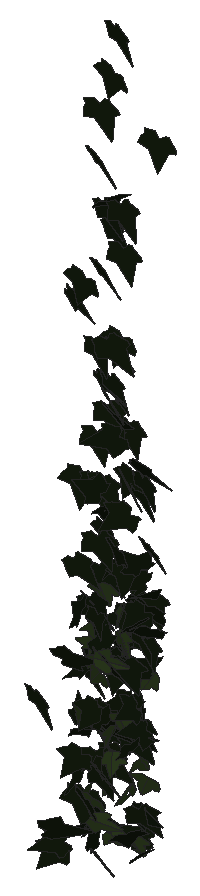
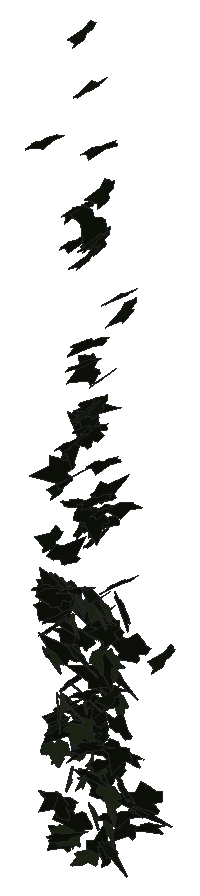
# SketchUp Ruby script. Lengths in inches.
U = 1.inch
M = Sketchup.active_model
def pt(a) = Geom::Point3d.new(a.map { |v| v * U })
def face(e, loops, mat)
  f = e.add_face(loops[0].map { |a| pt(a) })
  loops[1..].each { |l| e.add_face(l.map { |a| pt(a) }).erase! }
  f.material = f.back_material = mat if mat
  f
end
# faces: each face lists its corners as indices into pts; further lists are holes
def faces(e, pts, list, mat = nil) = list.each { |f| face(e, (f[0].is_a?(Array) ? f : [f]).map { |l| l.map { |i| pts[i] } }, mat) }
# xy, xz, yz: faces in a plane at the given z, y or x. An outline is a flat list of corners, or four numbers for a rectangle; further outlines are holes
def ring(l) = l.size == 4 ? [[l[0], l[1]], [l[2], l[1]], [l[2], l[3]], [l[0], l[3]]] : l.each_slice(2).to_a
def flat(e, list, mat, &to3) = list.each { |f| face(e, (f[0].is_a?(Array) ? f : [f]).map { |l| ring(l).map { |u, v| to3.(u, v) } }, mat) }
def xy(e, z, list, mat = nil) = flat(e, list, mat) { |x, y| [x, y, z] }
def xz(e, y, list, mat = nil) = flat(e, list, mat) { |x, z| [x, y, z] }
def yz(e, x, list, mat = nil) = flat(e, list, mat) { |y, z| [x, y, z] }
def lines(e, pts, list) = list.each { |a, b| e.add_line(pt(pts[a]), pt(pts[b])) }
# prism: a flat outline (further loops are holes) pulled along v
def prism(e, loops, v, mat = nil)
  f = face(e, loops, mat); d = Geom::Vector3d.new(v.map { |x| x * U })
  f.pushpull(f.normal.samedirection?(d) ? d.length : -d.length)
end
def box(e, o, s, mat = nil) = prism(e, [[o, [o[0] + s[0], o[1], o[2]], [o[0] + s[0], o[1] + s[1], o[2]], [o[0], o[1] + s[1], o[2]]]], [0, 0, s[2]], mat)
def at(x, y, z, deg = 0) = Geom::Transformation.translation(pt([x, y, z])) * Geom::Transformation.rotation(ORIGIN, Z_AXIS, deg.degrees)
def axes(o, x, y, z) = Geom::Transformation.new([*x, 0, *y, 0, *z, 0, *pt(o).to_a, 1])
def part(name) = M.definitions.add(name)
# library, detail: a bought-in or finely detailed component or shape, given as its bounding box
def library(name, o, s) = part(name).tap { |d| box(d.entities, o, s) }
def detail(e, o, s) = box(e.add_group.entities, o, s)
def put(e, d, t, mat = nil) = e.add_instance(d, t).tap { |i| i.material = mat if mat }
def group(e, t, mat = nil) = e.add_group.tap { |g| g.transformation = t; g.material = mat if mat }.entities
root = M.entities
M.materials.add("1026 AP 7946 SUNNY SIDE UP").color = [254, 231, 186]
M.materials.add("efeu1").color = [18, 25, 13]
M.materials.add("efeu2").color = [43, 57, 29]
c1 = part("ivyleaf_9")
p = [[1.54,2.16,1.25],[1.36,2.04,1.19],[-0.21,0.99,0.68],[-0.71,1.11,0.82],[-0.85,0.86,0.67],[-0.8,0.17,0.21],
  [-0.9,-0.01,0.1],[-0.67,-0.16,-0.02],[-0.08,-0.08,-0.05],[-0.03,-0.6,-0.4],[0.65,-0.88,-0.66],[0.83,-0.6,-0.49],
  [1.29,-0.42,-0.43],[1.8125,-0.07,-0.26],[1.21,0.44,0.15]]
faces(c1.entities,p,[[0,1,2,3,4,5,6,7,8,9,10,11,12,13,14]],"efeu1")
c2 = part("ivyleaf_10")
p = [[0,0.5,-0.03],[-0.0625,2.02,-0.43],[-0.19,2.01,-0.46],[-0.54,1.05,-0.29],[-0.52,0.625,-0.18],[-0.83,0.76,-0.28],
  [-1.16,0.64,-0.33],[-1.15,0.33,-0.24],[-0.77,-0.39,0.02],[-0.3,-0.51,0.16],[0.04,-0.48,0.23],[-0.02,2.01,-0.4375],
  [-0.06,2.01,-0.43],[0.04,-0.49,0.23],[0.67,-0.49,0.14],[1.38,0.36,-0.2],[1.375,0.51,-0.24],[0.81,0.65,-0.19],
  [0.62,0.59,-0.15],[0.6,1.09,-0.28],[0.5,1.23,-0.31]]
faces(c2.entities,p,[[0,1,2,3,4,5,6,7,8,9,10],[11,12,0,13,14,15,16,17,18,19,20]],"efeu2")
put(root,c1,axes([148.02,211.49,307.71],[-0.3468,-0.39947,-0.07155],[0.08263,0.04763,-0.46923],[0.63156,-0.22559,0.0221]),"1026 AP 7946 SUNNY SIDE UP")
put(root,c1,axes([148.12,211.17,296.1],[0.2283,0.3421,0.04637],[0.05922,0.03071,-0.38197],[-0.53891,0.1483,-0.02233]),"1026 AP 7946 SUNNY SIDE UP")
put(root,c1,axes([148.43,211.57,291.55],[-0.32957,0.32893,-0.01711],[-0.01222,-0.02684,-0.40138],[-0.51788,-0.20869,0.02037]),"1026 AP 7946 SUNNY SIDE UP")
put(root,c1,axes([148.27,210.93,294.23],[-0.39626,0.1337,-0.24009],[0.2906,-0.14709,-0.29271],[-0.30808,-0.31071,0.0327]),"1026 AP 7946 SUNNY SIDE UP")
put(root,c1,axes([148.47,211.86,300.53],[0.2781,-0.0272,-0.37505],[-0.57357,-0.02467,-0.18088],[-0.0163,0.40385,-0.03393]),"1026 AP 7946 SUNNY SIDE UP")
put(root,c2,axes([148.45,211.59,292.53],[0.30772,-0.23415,-0.22991],[-0.18469,0.18993,-0.31216],[0.47236,0.2268,0.02772]),"1026 AP 7946 SUNNY SIDE UP")
put(root,c1,axes([148.4,210.83,296.7],[0.37132,-0.08,0.31455],[-0.19132,0.32929,0.18747],[-0.45871,-0.2021,0.17644]),"1026 AP 7946 SUNNY SIDE UP")
put(root,c1,axes([148.01,210.98,303.96],[0.22055,-0.35797,-0.20662],[0.04313,0.21761,-0.38299],[0.64221,0.10832,0.09668]),"1026 AP 7946 SUNNY SIDE UP")
put(root,c1,axes([148.04,210.58,316.57],[0.50068,-0.29251,-0.15557],[-0.13487,0.12673,-0.44336],[0.4985,0.32807,0.03629]),"1026 AP 7946 SUNNY SIDE UP")
put(root,c1,axes([148.23,211.31,293.03],[-0.31586,-0.4262,-0.08847],[0.07842,0.0687,-0.48472],[0.67836,-0.20639,0.01484]),"1026 AP 7946 SUNNY SIDE UP")
put(root,c1,axes([148.49,209.25,291.48],[-0.43927,-0.24623,0.10603],[-0.08854,-0.09332,-0.38279],[0.41105,-0.28323,0.03085]),"1026 AP 7946 SUNNY SIDE UP")
put(root,c2,axes([148.43,211.375,293.48],[0.06296,-0.38932,-0.05728],[-0.0047,0.05337,-0.40287],[0.61788,0.04008,0.00277]),"1026 AP 7946 SUNNY SIDE UP")
put(root,c1,axes([148.67,210.84,299.35],[-0.45934,0.25194,-0.06801],[0.0441,-0.07034,-0.39623],[-0.40772,-0.29144,0.03376]),"1026 AP 7946 SUNNY SIDE UP")
put(root,c2,axes([148.47,211.86,300.69],[-0.37739,-0.31995,-0.0014],[0.04429,-0.02169,-0.41054],[0.50114,-0.23902,0.03522]),"1026 AP 7946 SUNNY SIDE UP")
put(root,c2,axes([148.64,211.45,300.1],[-0.54408,-0.13297,0.1484],[-0.16304,-0.12561,-0.37481],[0.26264,-0.35344,0.07475]),"1026 AP 7946 SUNNY SIDE UP")
put(root,c1,axes([148.86,209.05,292],[-0.57488,-0.00113,0.14571],[-0.22122,-0.03782,-0.37515],[0.02311,-0.39019,0.03363]),"1026 AP 7946 SUNNY SIDE UP")
put(root,c1,axes([148.14,211.56,298.66],[0.31074,-0.32465,0.07864],[0.04766,-0.07303,-0.39178],[0.52291,0.19958,-0.01103]),"1026 AP 7946 SUNNY SIDE UP")
put(root,c1,axes([148.04,211.73,301.84],[0.48195,-0.28561,0.13461],[0.11778,-0.11316,-0.43113],[0.4807,0.31407,-0.02933]),"1026 AP 7946 SUNNY SIDE UP")
put(root,c1,axes([148.12,208.23,298.98],[0.28091,-0.42459,0.1275],[0.05226,-0.12281,-0.47497],[0.69452,0.18097,-0.01583]),"1026 AP 7946 SUNNY SIDE UP")
put(root,c1,axes([148.375,211.09,317.13],[-0.20298,-0.3874,0.21408],[0.03188,-0.22382,-0.41382],[0.69215,-0.1033,0.08184]),"1026 AP 7946 SUNNY SIDE UP")
put(root,c1,axes([148.92,210.14,302.25],[-0.23648,0.02892,-0.46874],[-0.62543,0.2262,0.15152],[0.35092,0.42265,-0.04583]),"1026 AP 7946 SUNNY SIDE UP")
put(root,c2,axes([148.49,212.05,302.71],[0.39773,-0.28468,0.10174],[0.07112,-0.09374,-0.39184],[0.46929,0.25548,-0.02684]),"1026 AP 7946 SUNNY SIDE UP")
put(root,c1,axes([148.7,210.41,295.41],[-0.5666,-0.15043,-0.03454],[0.067,-0.01755,-0.40097],[0.2326,-0.36139,0.03137]),"1026 AP 7946 SUNNY SIDE UP")
put(root,c1,axes([148.33,211.75,307.58],[0.03559,-0.4106,-0.0915],[0.02211,0.0873,-0.42271],[0.65943,0.01924,0.01911]),"1026 AP 7946 SUNNY SIDE UP")
put(root,c1,axes([148.53,210.09,291.93],[0.20788,0.26926,0.22379],[0.1634,0.1892,-0.3078],[-0.51729,0.16796,-0.00729]),"1026 AP 7946 SUNNY SIDE UP")
put(root,c1,axes([148.2,211.9,322.52],[0.44796,-0.35322,0.0717],[0.02404,-0.07935,-0.46636],[0.56619,0.28283,-0.03693]),"1026 AP 7946 SUNNY SIDE UP")
put(root,c1,axes([148.38,212.125,324.74],[-0.01978,-0.45164,-0.12101],[0.04719,0.11392,-0.46401],[0.73125,-0.01957,0.02667]),"1026 AP 7946 SUNNY SIDE UP")
put(root,c1,axes([148.41,211.82,313.78],[0.1123,-0.43319,0.01438],[0.00141,-0.01649,-0.45239],[0.68164,0.0714,-0.00144]),"1026 AP 7946 SUNNY SIDE UP")
put(root,c1,axes([148.53,211.73,309.71],[-0.0936,-0.40561,-0.11167],[0.04233,0.10324,-0.42157],[0.65788,-0.06435,0.01124]),"1026 AP 7946 SUNNY SIDE UP")
put(root,c1,axes([148.7,211.13,290.84],[-0.03648,-0.08423,0.40935],[0.30326,0.34853,0.08965],[-0.56292,0.19322,0.02177]),"1026 AP 7946 SUNNY SIDE UP")
put(root,c1,axes([149.03,211.98,303.47],[-0.33954,0.33116,-0.0353],[0.00291,-0.04188,-0.40694],[-0.5238,-0.2149,0.02062]),"1026 AP 7946 SUNNY SIDE UP")
put(root,c1,axes([148.59,211.9,300.75],[-0.07609,-0.30763,0.28979],[-0.01236,-0.28421,-0.32128],[0.6572,-0.04097,0.02751]),"1026 AP 7946 SUNNY SIDE UP")
put(root,c2,axes([148.83,212.08,293.39],[0.33532,-0.28954,-0.11551],[-0.07935,0.09988,-0.36942],[0.48079,0.21842,0.01959]),"1026 AP 7946 SUNNY SIDE UP")
put(root,c1,axes([148.43,211.45,302.08],[-0.18706,-0.13328,-0.39864],[0.59372,0.11774,-0.16099],[0.24532,-0.38657,0.08566]),"1026 AP 7946 SUNNY SIDE UP")
put(root,c1,axes([148.3,209.87,299.98],[0.14046,-0.07305,0.42356],[0.61345,-0.13649,-0.11299],[0.23591,0.39841,0.04163]),"1026 AP 7946 SUNNY SIDE UP")
put(root,c1,axes([148.31,208.85,292.45],[0.31391,0.07645,0.44212],[0.6705,0.06146,-0.21549],[-0.13906,0.46892,-0.04098]),"1026 AP 7946 SUNNY SIDE UP")
put(root,c1,axes([148.57,211.99,303.38],[0.26727,-0.34837,-0.19096],[-0.02463,0.1936,-0.39271],[0.61855,0.15824,0.06687]),"1026 AP 7946 SUNNY SIDE UP")
put(root,c2,axes([149.08,210.0625,297.63],[-0.52109,0.16773,0.13464],[-0.21786,0.01096,-0.37912],[-0.25242,-0.35572,0.04926]),"1026 AP 7946 SUNNY SIDE UP")
put(root,c1,axes([149.17,212.4,296.32],[-0.40869,-0.17373,0.29317],[-0.32956,-0.19708,-0.3212],[0.40943,-0.33206,0.03409]),"1026 AP 7946 SUNNY SIDE UP")
put(root,c2,axes([148.87,211.61,302.76],[-0.60877,0.00636,-0.08419],[0.12702,-0.03828,-0.39738],[-0.02218,-0.39384,0.03494]),"1026 AP 7946 SUNNY SIDE UP")
put(root,c1,axes([148.62,212.07,320.23],[0.27941,-0.42204,-0.05816],[-0.01888,0.05359,-0.47133],[0.66877,0.17784,0.01099]),"1026 AP 7946 SUNNY SIDE UP")
put(root,c1,axes([148.61,211.81,312.36],[0.47341,-0.29564,-0.08159],[-0.0395,0.08451,-0.43205],[0.47895,0.29919,0.04501]),"1026 AP 7946 SUNNY SIDE UP")
put(root,c1,axes([149.21,210.97,307.52],[-0.0249,0.05717,0.46104],[-0.5437,-0.28869,0.02372],[0.4549,-0.34191,0.05358]),"1026 AP 7946 SUNNY SIDE UP")
put(root,c1,axes([148.58,211.58,299.46],[0.12732,0.0256,0.43926],[0.64664,0.11213,-0.08677],[-0.18077,0.41913,-0.00098]),"1026 AP 7946 SUNNY SIDE UP")
put(root,c1,axes([149.33,212.03,294.95],[-0.5707,-0.01598,0.0646],[-0.0965,-0.0299,-0.37342],[0.03271,-0.36712,0.02544]),"1026 AP 7946 SUNNY SIDE UP")
put(root,c2,axes([148.98,210.74,300.01],[0.00046,-0.18847,-0.35531],[0.21647,0.32198,-0.17982],[0.57728,-0.12059,0.06772]),"1026 AP 7946 SUNNY SIDE UP")
put(root,c1,axes([148.93,211.15,295.24],[-0.10478,-0.36629,-0.16019],[0.08068,0.14632,-0.38199],[0.6192,-0.08105,0.02267]),"1026 AP 7946 SUNNY SIDE UP")
put(root,c2,axes([149.29,210.47,293.47],[-0.5535,0.0779,0.09418],[-0.14864,-0.00727,-0.37044],[-0.11565,-0.3635,0.02537]),"1026 AP 7946 SUNNY SIDE UP")
put(root,c1,axes([149.18,211.55,320.85],[0.27598,0.40214,0.10968],[0.03447,0.10397,-0.4509],[-0.65229,0.17564,0.02258]),"1026 AP 7946 SUNNY SIDE UP")
put(root,c1,axes([148.91,212.17,312.15],[0.2732,-0.42689,-0.03594],[-0.03587,0.02576,-0.47451],[0.67222,0.17487,-0.01071]),"1026 AP 7946 SUNNY SIDE UP")
put(root,c1,axes([149.1875,212.21,298.82],[-0.24431,-0.34726,0.00141],[0.02574,-0.01097,-0.39147],[0.54545,-0.15502,0.0191]),"1026 AP 7946 SUNNY SIDE UP")
put(root,c1,axes([148.94,212.11,319.39],[0.34312,-0.40016,-0.07073],[-0.03918,0.06201,-0.46913],[0.63661,0.21949,0.00925]),"1026 AP 7946 SUNNY SIDE UP")
put(root,c2,axes([149.05,212.01,291.16],[-0.23712,-0.21454,-0.25466],[0.37237,0.11454,-0.25182],[0.35317,-0.26481,0.09453]),"1026 AP 7946 SUNNY SIDE UP")
put(root,c1,axes([149.03,211.51,307.73],[0.05445,-0.36917,-0.20136],[0.02906,0.1952,-0.37938],[0.65465,0.02204,0.03359]),"1026 AP 7946 SUNNY SIDE UP")
put(root,c1,axes([148.97,211.34,296.26],[0.09033,-0.22297,0.35513],[0.12246,-0.33714,-0.23912],[0.63552,0.09666,-0.0044]),"1026 AP 7946 SUNNY SIDE UP")
put(root,c1,axes([148.95,211.91,314.07],[0.63773,-0.19321,-0.03274],[-0.06565,-0.01648,-0.46167],[0.30052,0.4064,-0.03137]),"1026 AP 7946 SUNNY SIDE UP")
put(root,c1,axes([149.48,211.33,306.83],[0.09873,0.4085,-0.09498],[-0.01646,-0.09401,-0.42631],[-0.65909,0.06354,-0.00358]),"1026 AP 7946 SUNNY SIDE UP")
put(root,c2,axes([149.64,210.48,299.45],[-0.45691,0.10833,0.25052],[-0.37698,0.04791,-0.31764],[-0.17993,-0.37547,0.02933]),"1026 AP 7946 SUNNY SIDE UP")
put(root,c1,axes([149.1,211.75,311.13],[-0.00875,-0.38174,-0.1997],[0.07344,0.19001,-0.39011],[0.66764,-0.0259,0.04029]),"1026 AP 7946 SUNNY SIDE UP")
put(root,c1,axes([149.1875,210.68,297.74],[0.02362,-0.34461,-0.26966],[-0.03078,0.25915,-0.35377],[0.6779,0.02377,-0.00667]),"1026 AP 7946 SUNNY SIDE UP")
put(root,c2,axes([149.42,211.84,294.66],[0.13742,-0.13139,-0.36606],[0.06529,0.36506,-0.12668],[0.591,-0.00978,0.09911]),"1026 AP 7946 SUNNY SIDE UP")
put(root,c1,axes([149.07,211.9,311.32],[0.17018,-0.28055,0.31759],[0.15598,-0.29371,-0.31136],[0.6385,0.14652,-0.00859]),"1026 AP 7946 SUNNY SIDE UP")
put(root,c1,axes([149.25,211.38,305.6],[-0.06436,-0.33836,0.25632],[0.02795,-0.25308,-0.35033],[0.66161,-0.02223,0.03973]),"1026 AP 7946 SUNNY SIDE UP")
put(root,c1,axes([149.24,210.89,301.86],[0.05522,-0.38461,0.0884],[-0.00356,-0.08853,-0.39826],[0.62038,0.03373,-0.01016]),"1026 AP 7946 SUNNY SIDE UP")
put(root,c1,axes([149.27,211.47,296.41],[0.23561,-0.1991,-0.31417],[-0.12112,0.30377,-0.24243],[0.55819,0.14995,0.08]),"1026 AP 7946 SUNNY SIDE UP")
put(root,c1,axes([149.39,212.22,314.1875],[-0.23132,-0.40088,0.10837],[-0.01925,-0.10978,-0.43977],[0.65232,-0.1454,0.02545]),"1026 AP 7946 SUNNY SIDE UP")
put(root,c2,axes([149.4375,211.4,295.34],[-0.07112,0.25994,-0.27382],[0.02669,-0.26752,-0.27256],[-0.58563,-0.04376,0.02084]),"1026 AP 7946 SUNNY SIDE UP")
put(root,c1,axes([150.01,211.9,301.6],[-0.54729,0.16519,0.09326],[-0.19196,-0.0554,-0.38369],[-0.22464,-0.35511,0.10067]),"1026 AP 7946 SUNNY SIDE UP")
put(root,c1,axes([149.1,211.85,310.66],[0.09182,-0.17456,0.43265],[0.40086,-0.33927,-0.18334],[0.59395,0.25595,0.05686]),"1026 AP 7946 SUNNY SIDE UP")
put(root,c1,axes([149.72,210.23,298.02],[-0.49705,-0.23054,0.02018],[0.00189,-0.03699,-0.40205],[0.36399,-0.31463,0.02963]),"1026 AP 7946 SUNNY SIDE UP")
put(root,c1,axes([149.45,211.63,326.79],[-0.16654,-0.38276,0.26912],[0.04669,-0.27519,-0.40126],[0.7291,-0.06981,0.08717]),"1026 AP 7946 SUNNY SIDE UP")
put(root,c2,axes([149.58,211.92,296.79],[-0.53422,-0.11645,-0.11599],[0.20724,-0.04917,-0.35972],[0.14682,-0.35431,0.0857]),"1026 AP 7946 SUNNY SIDE UP")
put(root,c1,axes([149.6,210.72,290.56],[0.46947,-0.29558,-0.00792],[0.03936,0.01676,0.43185],[-0.4632,-0.29816,0.02866]),"1026 AP 7946 SUNNY SIDE UP")
put(root,c1,axes([149.36,209.93,293.8],[0.07572,-0.31024,0.33252],[0.16394,-0.30975,-0.32279],[0.68666,0.10816,0.0404]),"1026 AP 7946 SUNNY SIDE UP")
put(root,c1,axes([150.14,211.6875,300.31],[-0.40351,0.30391,0.05278],[-0.09787,0.01192,-0.40767],[-0.47417,-0.26108,0.03923]),"1026 AP 7946 SUNNY SIDE UP")
put(root,c1,axes([149.74,212.26,303.51],[-0.31337,-0.35263,0.03149],[0.06495,-0.06026,-0.41216],[0.55303,-0.19274,0.06625]),"1026 AP 7946 SUNNY SIDE UP")
put(root,c1,axes([150.16,209.93,297.65],[-0.01865,0.17594,0.39792],[-0.21673,0.36283,-0.17295],[-0.62971,-0.13009,0.04774]),"1026 AP 7946 SUNNY SIDE UP")
put(root,c1,axes([149.91,211.3,300.51],[0.36158,-0.33122,0.13683],[-0.05556,0.13832,0.41334],[-0.55949,-0.2278,0.04738]),"1026 AP 7946 SUNNY SIDE UP")
put(root,c1,axes([149.73,210.3,305.91],[-0.07485,-0.38237,-0.2301],[0.05406,0.21858,-0.39563],[0.69248,-0.05839,0.00601]),"1026 AP 7946 SUNNY SIDE UP")
put(root,c1,axes([149.67,211.05,314.68],[0.1099,-0.39347,-0.27182],[0.0869,0.26946,-0.40071],[0.73787,0.02687,0.08768]),"1026 AP 7946 SUNNY SIDE UP")
put(root,c1,axes([150.25,209.92,301.22],[-0.52411,0.23398,-0.17127],[-0.18101,0.12662,0.41876],[0.41476,0.35093,-0.03367]),"1026 AP 7946 SUNNY SIDE UP")
put(root,c1,axes([149.53,210.55,297.13],[0.5681,-0.02729,0.22385],[0.33089,-0.07385,-0.37019],[0.0962,0.41516,-0.04862]),"1026 AP 7946 SUNNY SIDE UP")
put(root,c1,axes([150.43,211.74,297.64],[-0.15132,0.24503,0.2832],[-0.26529,0.22164,-0.26441],[-0.51286,-0.18694,0.05321]),"1026 AP 7946 SUNNY SIDE UP")
put(root,c1,axes([149.88,212.16,310.36],[-0.00546,-0.43576,-0.04455],[0.00575,0.04074,-0.44868],[0.68816,-0.0038,0.0034]),"1026 AP 7946 SUNNY SIDE UP")
put(root,c1,axes([150.47,211.15,298.18],[-0.48927,0.21669,0.03964],[-0.08073,-0.00885,-0.38887],[-0.33616,-0.31326,0.03569]),"1026 AP 7946 SUNNY SIDE UP")
put(root,c1,axes([149.86,210.61,295.56],[0.24499,-0.26273,-0.35553],[-0.07952,0.35167,-0.29856],[0.67549,0.13668,0.0938]),"1026 AP 7946 SUNNY SIDE UP")
put(root,c1,axes([149.87,210.21,295.18],[-0.22455,-0.1129,-0.35893],[0.53928,0.08807,-0.17402],[0.1993,-0.36549,0.06647]),"1026 AP 7946 SUNNY SIDE UP")
put(root,c2,axes([150.28,211.46,296.23],[-0.41232,0.25335,0.08197],[-0.1186,0.03406,-0.37437],[-0.39965,-0.27148,0.02653]),"1026 AP 7946 SUNNY SIDE UP")
put(root,c1,axes([149.85,211.25,329.17],[0.30899,-0.43656,0.05918],[0.00891,-0.06311,-0.49312],[0.69283,0.19551,-0.02005]),"1026 AP 7946 SUNNY SIDE UP")
put(root,c1,axes([150.55,211.2,306.87],[-0.57428,-0.17005,0.12481],[-0.14679,-0.08751,-0.41368],[0.29466,-0.37503,0.03717]),"1026 AP 7946 SUNNY SIDE UP")
put(root,c1,axes([149.86,210.04,293.12],[0.41458,-0.04761,-0.26831],[0.41344,0.08707,0.25859],[0.04517,-0.36004,0.09575]),"1026 AP 7946 SUNNY SIDE UP")
put(root,c1,axes([150.1,211.34,320.97],[0.08552,-0.44018,-0.16251],[-0.03791,0.15344,-0.456],[0.73295,0.0593,-0.00463]),"1026 AP 7946 SUNNY SIDE UP")
put(root,c2,axes([150.25,211.2,302.42],[0.30554,-0.28823,0.19602],[0.13872,-0.17159,-0.35853],[0.52652,0.21247,-0.01929]),"1026 AP 7946 SUNNY SIDE UP")
put(root,c2,axes([150.3,211.82,293.87],[-0.26569,0.30318,0.1855],[0.15856,-0.14779,0.35639],[0.52987,0.19625,-0.01364]),"1026 AP 7946 SUNNY SIDE UP")
put(root,c2,axes([150.38,210.38,297.17],[0.04168,-0.37559,0.13578],[0.05916,-0.13128,-0.38769],[0.62422,0.03752,0.02768]),"1026 AP 7946 SUNNY SIDE UP")
put(root,c1,axes([150.71,212.2,291.46],[-0.23286,-0.30558,-0.16114],[-0.12527,-0.13317,0.34881],[-0.52378,0.16771,-0.01178]),"1026 AP 7946 SUNNY SIDE UP")
put(root,c1,axes([149.99,209.92,318.85],[0.46089,-0.35545,0.05904],[0.01483,-0.06889,-0.47356],[0.56645,0.29101,-0.03565]),"1026 AP 7946 SUNNY SIDE UP")
put(root,c1,axes([150.31,211.77,308.33],[-0.19803,-0.33998,0.21011],[-0.03535,-0.20953,-0.37185],[0.62396,-0.11977,0.04561]),"1026 AP 7946 SUNNY SIDE UP")
put(root,c1,axes([150.82,211.875,303.48],[-0.43073,0.29438,0.07535],[-0.12221,0.02484,-0.41212],[-0.46038,-0.28201,0.0389]),"1026 AP 7946 SUNNY SIDE UP")
put(root,c1,axes([150.66,210.37,310.89],[-0.05666,-0.20795,-0.41714],[-0.01906,-0.40442,0.21334],[-0.71384,0.0273,0.02741]),"1026 AP 7946 SUNNY SIDE UP")
put(root,c1,axes([150.57,211.05,292.06],[0.24165,0.41223,-0.04426],[-0.009,-0.0462,-0.45337],[-0.65204,0.15341,-0.01014]),"1026 AP 7946 SUNNY SIDE UP")
put(root,c2,axes([150.42,211.67,291.54],[-0.51915,-0.04325,-0.15041],[0.23183,-0.00605,-0.34225],[0.05833,-0.36085,0.02163]),"1026 AP 7946 SUNNY SIDE UP")
put(root,c1,axes([150.43,212.23,296.8125],[-0.02715,0.18118,0.4215],[-0.07212,-0.40698,0.18176],[0.69841,-0.03498,0.03515]),"1026 AP 7946 SUNNY SIDE UP")
put(root,c2,axes([150.5,211.25,301.19],[0.32407,-0.2923,0.18592],[0.14252,-0.15873,-0.36904],[0.52244,0.22462,-0.01465]),"1026 AP 7946 SUNNY SIDE UP")
put(root,c1,axes([150.84,211.58,304.33],[0.12879,0.08883,0.41015],[-0.58286,-0.15208,0.11277],[0.26589,-0.37641,0.04854]),"1026 AP 7946 SUNNY SIDE UP")
put(root,c1,axes([150.41,210.72,305.38],[-0.0518,-0.24272,0.36053],[0.05521,-0.35273,-0.24971],[0.66919,0.01031,0.04851]),"1026 AP 7946 SUNNY SIDE UP")
put(root,c1,axes([150.4375,211.07,319.18],[-0.0239,-0.45965,-0.07896],[-0.00812,0.07424,-0.47329],[0.73203,-0.01419,-0.00783]),"1026 AP 7946 SUNNY SIDE UP")
put(root,c2,axes([150.27,209.47,293.32],[-0.20354,-0.08134,-0.37778],[0.5525,0.10951,-0.15235],[0.20676,-0.37269,0.03521]),"1026 AP 7946 SUNNY SIDE UP")
put(root,c2,axes([150.59,210.11,296.11],[0.2571,0.34959,-0.09451],[-0.03823,-0.09201,-0.39776],[-0.56782,0.16448,-0.01601]),"1026 AP 7946 SUNNY SIDE UP")
put(root,c2,axes([150.77,211.63,297.76],[0.07348,-0.25905,-0.29774],[-0.063,0.28483,-0.2694],[0.60528,0.06109,0.0081]),"1026 AP 7946 SUNNY SIDE UP")
put(root,c1,axes([150.55,212.27,301.99],[-0.11098,-0.38637,0.04183],[-0.00087,-0.0434,-0.40481],[0.61125,-0.07021,0.00702]),"1026 AP 7946 SUNNY SIDE UP")
put(root,c1,axes([150.48,212.33,296.78],[-0.012,-0.34469,0.17944],[0.07551,-0.17565,-0.35301],[0.60396,0.01511,0.0477]),"1026 AP 7946 SUNNY SIDE UP")
put(root,c1,axes([150.34,209.76,295.36],[0.20858,-0.2932,0.28714],[0.23248,-0.23978,-0.33176],[0.59404,0.19678,0.02901]),"1026 AP 7946 SUNNY SIDE UP")
put(root,c1,axes([150.32,212.05,308.71],[0.59498,-0.12945,0.15257],[0.21932,-0.05207,-0.41228],[0.21931,0.40326,-0.00162]),"1026 AP 7946 SUNNY SIDE UP")
put(root,c1,axes([150.71,211.35,296.49],[-0.00336,-0.25291,-0.33451],[0.01574,0.32314,-0.25863],[0.6452,-0.0092,0.00457]),"1026 AP 7946 SUNNY SIDE UP")
put(root,c1,axes([150.98,211.08,298.08],[-0.20212,-0.20728,0.31517],[-0.21014,-0.27725,-0.25202],[0.54339,-0.18432,0.01977]),"1026 AP 7946 SUNNY SIDE UP")
put(root,c2,axes([150.91,211.54,295.45],[-0.10983,-0.31289,-0.23333],[0.13781,0.20948,-0.32732],[0.58983,-0.10721,0.03303]),"1026 AP 7946 SUNNY SIDE UP")
put(root,c1,axes([150.77,211.4,296.47],[0.50193,0.20052,0.04884],[0.07171,0.01435,-0.38807],[-0.31555,0.32223,-0.01049]),"1026 AP 7946 SUNNY SIDE UP")
put(root,c1,axes([150.65,211.77,307.78],[0.26264,-0.37187,0.09747],[0.0393,-0.09473,-0.42021],[0.6029,0.16817,-0.01507]),"1026 AP 7946 SUNNY SIDE UP")
put(root,c1,axes([150.93,211.3125,291.03],[0.21699,0.2228,0.2634],[0.14244,0.24039,-0.26608],[-0.51232,0.1612,0.03758]),"1026 AP 7946 SUNNY SIDE UP")
put(root,c1,axes([150.46,209.64,300.78],[0.39266,-0.28255,0.30317],[0.28154,-0.23621,-0.38943],[0.57843,0.30678,-0.01625]),"1026 AP 7946 SUNNY SIDE UP")
put(root,c1,axes([150.7,211.83,302.59],[0.54275,0.22399,0.03604],[-0.0752,0.012,0.42235],[0.34814,-0.34661,0.03504]),"1026 AP 7946 SUNNY SIDE UP")
put(root,c1,axes([150.53,211.83,292.79],[0.28213,-0.12111,-0.33738],[0.54682,0.08644,0.16421],[0.03611,-0.36266,0.14932]),"1026 AP 7946 SUNNY SIDE UP")
put(root,c2,axes([150.84,210.42,301.69],[-0.40387,0.1484,-0.2719],[0.23514,-0.23997,-0.28941],[-0.41533,-0.28017,0.10055]),"1026 AP 7946 SUNNY SIDE UP")
put(root,c1,axes([150.68,211.4,299.59],[-0.18875,0.0257,0.41372],[0.61284,-0.0963,0.12584],[0.15661,0.40779,0.00617]),"1026 AP 7946 SUNNY SIDE UP")
put(root,c2,axes([150.66,209.31,300.99],[0.00696,0.05155,0.41115],[0.49825,0.2451,-0.03482],[-0.38928,0.31463,-0.03722]),"1026 AP 7946 SUNNY SIDE UP")
put(root,c1,axes([151.37,210.18,296.6],[-0.06047,0.35479,0.2007],[-0.08673,0.18725,-0.3652],[-0.62897,-0.05993,0.03107]),"1026 AP 7946 SUNNY SIDE UP")
put(root,c1,axes([150.83,211.64,293.03],[-0.13434,-0.17051,-0.3505],[0.26756,0.29367,-0.19448],[0.53373,-0.19014,0.00927]),"1026 AP 7946 SUNNY SIDE UP")
put(root,c1,axes([151.36,211.42,302.76],[0.34287,0.13607,-0.38084],[-0.47469,-0.2151,-0.26571],[-0.3997,0.37218,-0.01113]),"1026 AP 7946 SUNNY SIDE UP")
put(root,c1,axes([151.1875,211.45,296.96],[0.09203,-0.30477,-0.31963],[0.10805,-0.30088,0.31786],[-0.6733,-0.08994,0.00732]),"1026 AP 7946 SUNNY SIDE UP")
put(root,c1,axes([150.9,210.6,300.37],[-0.27444,-0.26431,-0.29574],[0.29433,0.21736,-0.32383],[0.5364,-0.2545,0.02638]),"1026 AP 7946 SUNNY SIDE UP")
put(root,c1,axes([150.94,211.67,301.23],[0.08817,-0.3996,0.02973],[-0.00267,-0.03167,-0.41583],[0.63022,0.05577,-0.00592]),"1026 AP 7946 SUNNY SIDE UP")
put(root,c1,axes([151.52,211.43,301.75],[0.01511,0.27596,-0.29397],[-0.25785,-0.25878,-0.26358],[-0.57038,0.12429,0.11137]),"1026 AP 7946 SUNNY SIDE UP")
put(root,c1,axes([151.33,210.65,308.15],[0.23378,-0.38042,0.22052],[-0.03783,0.2209,0.41873],[-0.68699,-0.14162,0.05198]),"1026 AP 7946 SUNNY SIDE UP")
put(root,c2,axes([151.16,209.92,294.34],[0.10816,-0.35708,0.16121],[-0.00122,0.16083,0.37451],[-0.6143,-0.06319,0.02764]),"1026 AP 7946 SUNNY SIDE UP")
put(root,c1,axes([151.46,211,302.75],[-0.61513,-0.04852,-0.06951],[0.11178,-0.0297,-0.40441],[0.06701,-0.39582,0.0365]),"1026 AP 7946 SUNNY SIDE UP")
put(root,c1,axes([151.45,210.51,302.36],[0.05778,0.41903,0.00811],[0.00638,0.00516,-0.43329],[-0.6589,0.0368,-0.00349]),"1026 AP 7946 SUNNY SIDE UP")
put(root,c1,axes([151.09,211.86,302.96],[-0.16223,-0.35909,-0.21916],[0.1714,0.1862,-0.38082],[0.63181,-0.14272,0.04704]),"1026 AP 7946 SUNNY SIDE UP")
put(root,c1,axes([150.96,211.95,305.23],[0.28435,-0.31476,0.17593],[0.13557,-0.14948,-0.37484],[0.5479,0.20034,0.00145]),"1026 AP 7946 SUNNY SIDE UP")
put(root,c1,axes([151.09,211.52,308.55],[0.17994,-0.39826,0.08111],[0.02511,-0.07967,-0.4273],[0.63854,0.11536,-0.00605]),"1026 AP 7946 SUNNY SIDE UP")
put(root,c1,axes([151.1875,211.68,301.02],[0.02881,-0.41004,0.00574],[-0.00205,-0.00797,-0.42289],[0.64487,0.01829,-0.0016]),"1026 AP 7946 SUNNY SIDE UP")
put(root,c2,axes([151.61,211.15,294.91],[-0.54916,-0.04405,0.12231],[-0.17562,-0.05853,-0.36043],[0.09462,-0.36429,0.0409]),"1026 AP 7946 SUNNY SIDE UP")
put(root,c2,axes([151.5,211.53,299.56],[0.5108,-0.20029,-0.10384],[-0.15006,0.03484,-0.39243],[0.31816,0.338,-0.01839]),"1026 AP 7946 SUNNY SIDE UP")
put(root,c1,axes([151.28,212.29,324.08],[-0.16534,-0.45051,0.0197],[0.00801,-0.02345,-0.47661],[0.70916,-0.10477,0.00998]),"1026 AP 7946 SUNNY SIDE UP")
